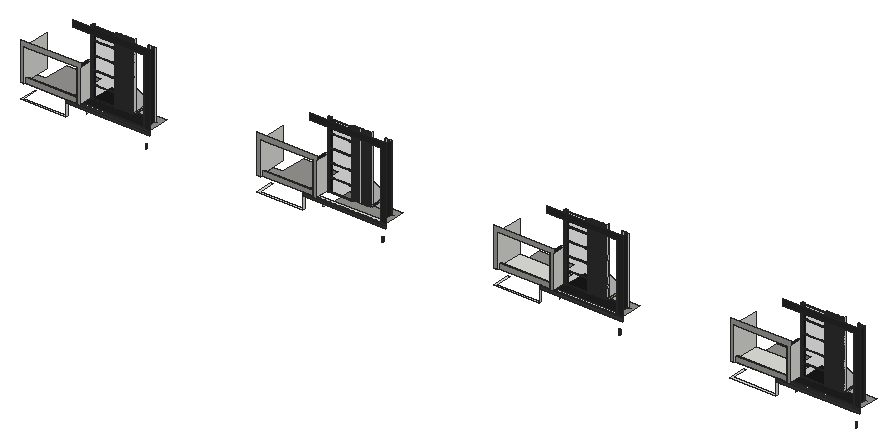
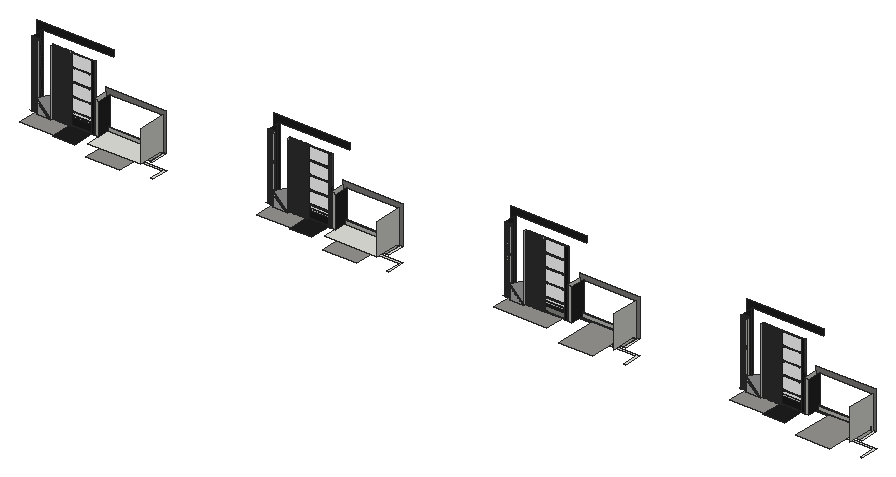
# SketchUp Ruby script. Lengths in inches.
U = 1.inch
M = Sketchup.active_model
def pt(a) = Geom::Point3d.new(a.map { |v| v * U })
def face(e, loops, mat)
  f = e.add_face(loops[0].map { |a| pt(a) })
  loops[1..].each { |l| e.add_face(l.map { |a| pt(a) }).erase! }
  f.material = f.back_material = mat if mat
  f
end
# faces: each face lists its corners as indices into pts; further lists are holes
def faces(e, pts, list, mat = nil) = list.each { |f| face(e, (f[0].is_a?(Array) ? f : [f]).map { |l| l.map { |i| pts[i] } }, mat) }
# xy, xz, yz: faces in a plane at the given z, y or x. An outline is a flat list of corners, or four numbers for a rectangle; further outlines are holes
def ring(l) = l.size == 4 ? [[l[0], l[1]], [l[2], l[1]], [l[2], l[3]], [l[0], l[3]]] : l.each_slice(2).to_a
def flat(e, list, mat, &to3) = list.each { |f| face(e, (f[0].is_a?(Array) ? f : [f]).map { |l| ring(l).map { |u, v| to3.(u, v) } }, mat) }
def xy(e, z, list, mat = nil) = flat(e, list, mat) { |x, y| [x, y, z] }
def xz(e, y, list, mat = nil) = flat(e, list, mat) { |x, z| [x, y, z] }
def yz(e, x, list, mat = nil) = flat(e, list, mat) { |y, z| [x, y, z] }
def lines(e, pts, list) = list.each { |a, b| e.add_line(pt(pts[a]), pt(pts[b])) }
# prism: a flat outline (further loops are holes) pulled along v
def prism(e, loops, v, mat = nil)
  f = face(e, loops, mat); d = Geom::Vector3d.new(v.map { |x| x * U })
  f.pushpull(f.normal.samedirection?(d) ? d.length : -d.length)
end
def box(e, o, s, mat = nil) = prism(e, [[o, [o[0] + s[0], o[1], o[2]], [o[0] + s[0], o[1] + s[1], o[2]], [o[0], o[1] + s[1], o[2]]]], [0, 0, s[2]], mat)
def at(x, y, z, deg = 0) = Geom::Transformation.translation(pt([x, y, z])) * Geom::Transformation.rotation(ORIGIN, Z_AXIS, deg.degrees)
def axes(o, x, y, z) = Geom::Transformation.new([*x, 0, *y, 0, *z, 0, *pt(o).to_a, 1])
def part(name) = M.definitions.add(name)
# library, detail: a bought-in or finely detailed component or shape, given as its bounding box
def library(name, o, s) = part(name).tap { |d| box(d.entities, o, s) }
def detail(e, o, s) = box(e.add_group.entities, o, s)
def put(e, d, t, mat = nil) = e.add_instance(d, t).tap { |i| i.material = mat if mat }
def group(e, t, mat = nil) = e.add_group.tap { |g| g.transformation = t; g.material = mat if mat }.entities
root = M.entities
M.materials.add("Aluminum_Polished").color = [83, 85, 85]
M.materials.add("Glass_Window_Neutral").color = [0, 0, 0]
M.materials["Glass_Window_Neutral"].alpha = 0.125
M.materials.add("[Carrera Marble]").color = [207, 207, 207]
M.materials.add("[Color M07]").color = [58, 58, 58]
M.materials.add("[Color M08]").color = [30, 30, 30]
M.materials.add("[Field Square Tile]").color = [211, 167, 108]
M.materials.add("[Granite Dark Gray]").color = [38, 37, 37]
M.materials.add("[Granite Light Gray]").color = [149, 148, 144]
M.materials.add("[Granite Tile]1").color = [68, 65, 63]
c1 = part("Group\#7")
xy(c1.entities,0,[[6,0,4.45,0.2,3,0.8,1.76,1.76,0.8,3,0.2,4.45,0,6,0.2,7.55,0.8,9,1.76,10.24,3,11.2,4.45,11.8,6,12,7.55,11.8,9,11.2,10.24,10.24,11.2,9,11.8,7.55,12,6,11.8,4.45,11.2,3,10.24,1.76,9,0.8,7.55,0.2]])
xy(c1.entities,37,[[6,0,7.55,0.2,9,0.8,10.24,1.76,11.2,3,11.8,4.45,12,6,11.8,7.55,11.2,9,10.24,10.24,9,11.2,7.55,11.8,6,12,4.45,11.8,3,11.2,1.76,10.24,0.8,9,0.2,7.55,0,6,0.2,4.45,0.8,3,1.76,1.76,3,0.8,4.45,0.2]],"[Granite Tile]1")
p = [[4.45,0.2,0],[6,0,0],[6,0,37],[4.45,0.2,37],[7.55,0.2,0],[7.55,0.2,37],
  [3,0.8,0],[3,0.8,37],[9,0.8,0],[9,0.8,37],[1.76,1.76,0],[1.76,1.76,37],
  [10.24,1.76,0],[10.24,1.76,37],[0.8,3,0],[0.8,3,37],[11.2,3,0],[11.2,3,37],
  [0.2,4.45,0],[0.2,4.45,37],[11.8,4.45,0],[11.8,4.45,37],[0,6,0],[0,6,37],
  [12,6,0],[12,6,37],[0.2,7.55,0],[0.2,7.55,37],[11.8,7.55,0],[11.8,7.55,37],
  [0.8,9,0],[0.8,9,37],[11.2,9,0],[11.2,9,37],[1.76,10.24,0],[1.76,10.24,37],
  [10.24,10.24,0],[10.24,10.24,37],[3,11.2,0],[3,11.2,37],[9,11.2,0],[9,11.2,37],
  [4.45,11.8,0],[4.45,11.8,37],[7.55,11.8,0],[7.55,11.8,37],[6,12,0],[6,12,37]]
faces(c1.entities,p,[[0,1,2,3],[1,4,5,2],[6,0,3,7],[4,8,9,5],[10,6,7,11],[8,12,13,9],[14,10,11,15],[12,16,17,13],
  [18,14,15,19],[16,20,21,17],[22,18,19,23],[20,24,25,21],[26,22,23,27],[24,28,29,25],[30,26,27,31],[28,32,33,29],
  [34,30,31,35],[32,36,37,33],[38,34,35,39],[36,40,41,37],[42,38,39,43],[40,44,45,41],[46,42,43,47],[44,46,47,45]],"[Granite Tile]1")
c2 = part("Group\#54")
box(c2.entities,[0,0,0],[2,1,28])
c3 = part("Group\#56")
p = [[0.11,0.32,0.14],[0.11,0.69,0.14]]
lines(c3.entities,p,[[0,1]])
g1 = group(c3.entities,at(0.11,0,0))
prism(g1,[[[0,0.24,0],[0,0.32,0.14],[0,0.24,0.27],[0,0.08,0.27],[0,0,0.14],[0,0.08,0]]],[-0.11,0,0])
c4 = part("Ver Glass Railing")
g2 = group(c4.entities,at(0,0,0),"Aluminum_Polished")
box(g2,[0,0,0],[2,185,2])
g3 = group(c4.entities,at(0,0,2),"Aluminum_Polished")
p = [[1.41,1,0],[1.41,36.8,0],[1.41,184,0],[1.29,184,0],[1.29,1,0],[1.29,36.8,0],
  [1.41,184,28],[1.29,184,28],[1.41,148.2,28],[1.29,148.2,28],[1.41,1,28],[1.29,1,28],
  [1.29,111.4,28],[1.29,111.4,0],[1.41,111.4,0],[1.41,111.4,28],[1.29,110.4,0],[1.29,110.4,28],
  [1.41,110.4,28],[1.41,110.4,0],[1.29,74.6,28],[1.29,74.6,0],[1.41,74.6,0],[1.41,74.6,28],
  [1.29,73.6,0],[1.29,73.6,28],[1.41,73.6,28],[1.41,73.6,0],[1.29,148.2,0],[1.41,148.2,0],
  [1.29,147.2,0],[1.29,147.2,28],[1.41,147.2,28],[1.41,147.2,0],[1.29,37.8,28],[1.29,37.8,0],
  [1.41,37.8,0],[1.41,37.8,28],[1.29,36.8,28],[1.41,36.8,28]]
lines(g3,p,[[0,1],[2,3],[4,5],[6,7],[6,8],[7,9],[10,11],[2,6],[3,7],[0,4],[11,4],[10,0],
  [12,13],[14,15],[16,17],[18,19],[20,21],[22,23],[24,25],[26,27],[27,22],[24,21],[23,26],[20,25],
  [9,28],[29,8],[30,31],[32,33],[33,29],[30,28],[8,32],[9,31],[34,35],[36,37],[5,38],[39,1],
  [1,36],[5,35],[37,39],[14,33],[19,14],[22,19],[36,27],[13,30],[16,13],[21,16],[35,24],[15,18],
  [12,17],[29,2],[28,3],[18,23],[32,15],[17,20],[31,12],[26,37],[25,34],[34,38],[39,10],[38,11]])
g4 = group(g3,at(1.79,1,0))
box(g4,[-0.5,0,0],[0.125,183,28],"Glass_Window_Neutral")
g5 = group(g3,at(0,184,28))
box(g5,[0,-184,0],[2.5,185,1])
put(g3,c2,axes([2,185,28],[-1,0,0],[0,-1,0],[0,0,-1]))
put(g3,c2,axes([2,1,28],[-1,0,0],[0,-1,0],[0,0,-1]))
put(g3,c2,axes([2,111.4,28],[-1,0,0],[0,-1,0],[0,0,-1]))
put(g3,c2,axes([2,74.6,28],[-1,0,0],[0,-1,0],[0,0,-1]))
g6 = group(g3,at(2,148.2,28))
box(g6,[-2,-1,-28],[2,1,28])
put(g3,c2,axes([2,37.8,28],[-1,0,0],[0,-1,0],[0,0,-1]))
put(g3,c3,at(1.17,146.31,24.26))
put(g3,c3,axes([1.17,148.89,24.54],[1,0,0],[0,-1,0],[0,0,-1]))
put(g3,c3,axes([1.17,148.89,4.79],[1,0,0],[0,-1,0],[0,0,-1]))
put(g3,c3,at(1.17,146.31,4.51))
put(g3,c3,at(1.17,109.51,4.51))
put(g3,c3,axes([1.17,112.09,4.79],[1,0,0],[0,-1,0],[0,0,-1]))
put(g3,c3,axes([1.17,112.09,24.54],[1,0,0],[0,-1,0],[0,0,-1]))
put(g3,c3,at(1.17,109.51,24.26))
put(g3,c3,axes([1.17,75.29,24.54],[1,0,0],[0,-1,0],[0,0,-1]))
put(g3,c3,at(1.17,72.71,4.51))
put(g3,c3,axes([1.17,75.29,4.79],[1,0,0],[0,-1,0],[0,0,-1]))
put(g3,c3,at(1.17,72.71,24.26))
put(g3,c3,axes([1.17,38.49,24.54],[1,0,0],[0,-1,0],[0,0,-1]))
put(g3,c3,at(1.17,35.91,4.51))
put(g3,c3,axes([1.17,38.49,4.79],[1,0,0],[0,-1,0],[0,0,-1]))
put(g3,c3,at(1.17,35.91,24.26))
xy(root,72.4375,[[218.97,457.5625,388.78,457.5625,388.78,465.32,225.79,465.32,225.79,523.18,218.97,523.18],[1097.72,457.5625,1267.53,457.5625,1267.53,465.32,1104.54,465.32,1104.54,523.18,1097.72,523.18],[1976.47,457.5625,2146.28,457.5625,2146.28,465.32,1983.29,465.32,1983.29,523.18,1976.47,523.18],[2855.22,457.5625,3025.03,457.5625,3025.03,465.32,2862.04,465.32,2862.04,523.18,2855.22,523.18]])
xy(root,118.38,[[463.7,458.5,481.29,465.32],[1342.45,458.5,1360.04,465.32],[2221.2,458.5,2238.79,465.32],[3099.95,458.5,3117.54,465.32]])
xy(root,118.38,[[481.29,458.5,678.9,561.06],[1360.04,458.5,1557.65,561.06],[2238.79,458.5,2436.4,561.06],[3117.54,458.5,3315.15,561.06]],"[Granite Light Gray]")
xy(root,128.5,[[218.97,458.5,225.79,523.18],[388.78,458.5,399.95,463.25],[399.95,458.5,427.1,463.25],[427.1,458.5,427.1,463.25,399.95,463.25,399.95,465.32,678.9,465.32,678.9,458.5],[1097.72,458.5,1104.54,523.18],
  [1267.53,458.5,1278.7,463.25],[1278.7,458.5,1305.85,463.25],[1305.85,458.5,1305.85,463.25,1278.7,463.25,1278.7,465.32,1557.65,465.32,1557.65,458.5],[1976.47,458.5,1983.29,523.18],[2146.28,458.5,2157.45,463.25],
  [2157.45,458.5,2184.6,463.25],[2184.6,458.5,2184.6,463.25,2157.45,463.25,2157.45,465.32,2436.4,465.32,2436.4,458.5],[2855.22,458.5,2862.04,523.18],[3025.03,458.5,3036.2,463.25],[3036.2,458.5,3063.35,463.25],
  [3063.35,458.5,3063.35,463.25,3036.2,463.25,3036.2,465.32,3315.15,465.32,3315.15,458.5]])
xy(root,128.5,[[228.78,458.5,228.78,523.18,262.66,523.18,262.66,619.06,388.78,619.06,388.78,463.25,232.96,463.25,232.96,458.5],[1107.53,458.5,1107.53,523.18,1141.41,523.18,1141.41,619.06,1267.53,619.06,1267.53,463.25,1111.71,463.25,1111.71,458.5],[1986.28,458.5,1986.28,523.18,2020.16,523.18,2020.16,619.06,2146.28,619.06,2146.28,463.25,1990.46,463.25,1990.46,458.5],[2865.03,458.5,2865.03,523.18,2898.91,523.18,2898.91,619.06,3025.03,619.06,3025.03,463.25,2869.21,463.25,2869.21,458.5]],"[Granite Light Gray]")
xy(root,134.5,[[442.35,458.5,676.54,458.5,676.54,468.31,444.78,468.31,444.78,511.08,442.35,511.08],[1321.1,458.5,1555.29,458.5,1555.29,468.31,1323.53,468.31,1323.53,511.08,1321.1,511.08],[2199.85,458.5,2434.04,458.5,2434.04,468.31,2202.28,468.31,2202.28,511.08,2199.85,511.08],[3078.6,458.5,3312.79,458.5,3312.79,468.31,3081.03,468.31,3081.03,511.08,3078.6,511.08],[1990.46,468.31,2184.6,561.05],
  [2869.21,468.31,3063.35,561.05],[534.46,508.33,539.88,511.08],[541.08,508.33,546.51,511.08],[547.71,508.33,553.13,511.08],[554.33,508.33,559.76,511.08],
  [560.96,508.33,566.38,511.08],[567.58,508.33,573.01,511.08],[574.21,508.33,579.63,511.08],[580.83,508.33,586.26,511.08],[587.46,508.33,592.88,511.08],
  [594.08,508.33,599.51,511.08],[653.06,508.33,658.48,511.08],[659.68,508.33,665.11,511.08],[666.31,508.33,671.73,511.08],[672.56,508.33,676.54,511.08],
  [676.54,508.33,677.98,511.08],[1413.21,508.33,1418.63,511.08],[1419.83,508.33,1425.26,511.08],[1426.46,508.33,1431.88,511.08],[1433.08,508.33,1438.51,511.08],
  [1439.71,508.33,1445.13,511.08],[1446.33,508.33,1451.76,511.08],[1459.58,508.33,1465.01,511.08],[1466.21,508.33,1471.63,511.08],[1472.83,508.33,1478.26,511.08],
  [1531.81,508.33,1537.23,511.08],[1538.43,508.33,1543.86,511.08],[1545.06,508.33,1550.48,511.08],[1555.29,508.33,1556.73,511.08],[2291.96,508.33,2297.38,511.08],
  [2298.58,508.33,2304.01,511.08],[2305.21,508.33,2310.63,511.08],[2311.83,508.33,2317.26,511.08],[2318.46,508.33,2323.88,511.08],[2325.08,508.33,2330.51,511.08],
  [2331.71,508.33,2337.13,511.08],[2338.33,508.33,2343.76,511.08],[2344.96,508.33,2350.38,511.08],[2351.58,508.33,2357.01,511.08],[2410.56,508.33,2415.98,511.08],
  [2417.18,508.33,2422.61,511.08],[2423.81,508.33,2429.23,511.08],[2430.06,508.33,2434.04,511.08],[2434.04,508.33,2435.48,511.08],[3170.71,508.33,3176.13,511.08],
  [3177.33,508.33,3182.76,511.08],[3183.96,508.33,3189.38,511.08],[3190.58,508.33,3196.01,511.08],[3197.21,508.33,3202.63,511.08],[3203.83,508.33,3209.26,511.08],
  [3210.46,508.33,3215.88,511.08],[3217.08,508.33,3222.51,511.08],[3223.71,508.33,3229.13,511.08],[3230.33,508.33,3235.76,511.08],[3289.31,508.33,3294.73,511.08],
  [3295.93,508.33,3301.36,511.08],[3302.56,508.33,3307.98,511.08],[3308.81,508.33,3312.79,511.08],[3312.79,508.33,3314.23,511.08]])
xy(root,134.5,[[444.78,468.31,676.54,468.31,676.54,508.33,672.56,508.33,672.56,511.08,671.73,511.08,671.73,508.33,666.31,508.33,666.31,511.08,665.11,511.08,665.11,508.33,659.68,508.33,659.68,511.08,658.48,511.08,658.48,508.33,653.06,508.33,653.06,518.65,605.1875,518.65,605.1875,513.52,599.51,513.52,599.51,508.33,594.08,508.33,594.08,511.08,592.88,511.08,592.88,508.33,587.46,508.33,587.46,511.08,586.26,511.08,586.26,508.33,580.83,508.33,580.83,511.08,579.63,511.08,579.63,508.33,574.21,508.33,574.21,511.08,573.01,511.08,573.01,508.33,567.58,508.33,567.58,511.08,566.38,511.08,566.38,508.33,560.96,508.33,560.96,511.08,559.76,511.08,559.76,508.33,554.33,508.33,554.33,511.08,553.13,511.08,553.13,508.33,547.71,508.33,547.71,511.08,546.51,511.08,546.51,508.33,541.08,508.33,541.08,511.08,539.88,511.08,539.88,508.33,534.46,508.33,534.46,589.83,453.7,589.83,453.7,511.08,444.78,511.08],[2202.28,468.31,2434.04,468.31,2434.04,508.33,2430.06,508.33,2430.06,511.08,2429.23,511.08,2429.23,508.33,2423.81,508.33,2423.81,511.08,2422.61,511.08,2422.61,508.33,2417.18,508.33,2417.18,511.08,2415.98,511.08,2415.98,508.33,2410.56,508.33,2410.56,518.65,2362.6875,518.65,2362.6875,513.52,2357.01,513.52,2357.01,508.33,2351.58,508.33,2351.58,511.08,2350.38,511.08,2350.38,508.33,2344.96,508.33,2344.96,511.08,2343.76,511.08,2343.76,508.33,2338.33,508.33,2338.33,511.08,2337.13,511.08,2337.13,508.33,2331.71,508.33,2331.71,511.08,2330.51,511.08,2330.51,508.33,2325.08,508.33,2325.08,511.08,2323.88,511.08,2323.88,508.33,2318.46,508.33,2318.46,511.08,2317.26,511.08,2317.26,508.33,2311.83,508.33,2311.83,511.08,2310.63,511.08,2310.63,508.33,2305.21,508.33,2305.21,511.08,2304.01,511.08,2304.01,508.33,2298.58,508.33,2298.58,511.08,2297.38,511.08,2297.38,508.33,2291.96,508.33,2291.96,589.83,2211.2,589.83,2211.2,511.08,2202.28,511.08],[3081.03,468.31,3312.79,468.31,3312.79,508.33,3308.81,508.33,3308.81,511.08,3307.98,511.08,3307.98,508.33,3302.56,508.33,3302.56,511.08,3301.36,511.08,3301.36,508.33,3295.93,508.33,3295.93,511.08,3294.73,511.08,3294.73,508.33,3289.31,508.33,3289.31,518.65,3241.4375,518.65,3241.4375,513.52,3235.76,513.52,3235.76,508.33,3230.33,508.33,3230.33,511.08,3229.13,511.08,3229.13,508.33,3223.71,508.33,3223.71,511.08,3222.51,511.08,3222.51,508.33,3217.08,508.33,3217.08,511.08,3215.88,511.08,3215.88,508.33,3210.46,508.33,3210.46,511.08,3209.26,511.08,3209.26,508.33,3203.83,508.33,3203.83,511.08,3202.63,511.08,3202.63,508.33,3197.21,508.33,3197.21,511.08,3196.01,511.08,3196.01,508.33,3190.58,508.33,3190.58,511.08,3189.38,511.08,3189.38,508.33,3183.96,508.33,3183.96,511.08,3182.76,511.08,3182.76,508.33,3177.33,508.33,3177.33,511.08,3176.13,511.08,3176.13,508.33,3170.71,508.33,3170.71,589.83,3089.95,589.83,3089.95,511.08,3081.03,511.08]],"[Color M08]")
xz(root,458.5,[[388.78,118.38,698.16,128.5],[1267.53,118.38,1576.91,128.5],[2146.28,118.38,2455.66,128.5],[3025.03,118.38,3334.41,128.5],[442.35,128.5,698.16,134.5],
  [1321.1,128.5,1576.91,134.5],[2199.85,128.5,2455.66,134.5],[3078.6,128.5,3334.41,134.5]],"[Color M07]")
xz(root,458.5,[[676.54,134.5,698.16,134.5,698.16,403.8125,414.98,403.8125,414.98,380.5,676.54,380.5],[1555.29,134.5,1576.91,134.5,1576.91,403.8125,1293.73,403.8125,1293.73,380.5,1555.29,380.5],[2434.04,134.5,2455.66,134.5,2455.66,403.8125,2172.48,403.8125,2172.48,380.5,2434.04,380.5],[3312.79,134.5,3334.41,134.5,3334.41,403.8125,3051.23,403.8125,3051.23,380.5,3312.79,380.5]],"[Granite Dark Gray]")
xz(root,458.5,[[218.97,128.5,232.96,128.5,232.96,251.5,427.1,251.5,427.1,128.5,442.35,128.5,442.35,270.8125,218.97,270.8125],[1097.72,128.5,1111.71,128.5,1111.71,251.5,1305.85,251.5,1305.85,128.5,1321.1,128.5,1321.1,270.8125,1097.72,270.8125],[1976.47,128.5,1990.46,128.5,1990.46,251.5,2184.6,251.5,2184.6,128.5,2199.85,128.5,2199.85,270.8125,1976.47,270.8125],[2855.22,128.5,2869.21,128.5,2869.21,251.5,3063.35,251.5,3063.35,128.5,3078.6,128.5,3078.6,270.8125,2855.22,270.8125]],"[Granite Light Gray]")
xz(root,463.25,[[232.96,128.5,427.1,147.6875],[1111.71,128.5,1305.85,147.6875],[1990.46,128.5,2184.6,147.6875],[2869.21,128.5,3063.35,147.6875]],"[Granite Light Gray]")
xz(root,468.31,[[232.96,134.5,427.1,147.6875],[1111.71,134.5,1305.85,147.6875],[1990.46,134.5,2184.6,147.6875],[2869.21,134.5,3063.35,147.6875]])
xz(root,508.33,[[672.56,134.5,677.98,380.5],[2430.06,134.5,2435.48,380.5],[3308.81,134.5,3314.23,380.5]],"[Field Square Tile]")
xz(root,508.33,[[534.46,134.5,539.88,380.5],[541.08,134.5,546.51,380.5],[547.71,134.5,553.13,380.5],[554.33,134.5,559.76,380.5],[560.96,134.5,566.38,380.5],
  [567.58,134.5,573.01,380.5],[574.21,134.5,579.63,380.5],[580.83,134.5,586.26,380.5],[587.46,134.5,592.88,380.5],[594.08,134.5,599.51,380.5],
  [653.06,134.5,658.48,380.5],[659.68,134.5,665.11,210.79],[666.31,134.5,671.73,380.5],[1413.21,134.5,1418.63,380.5],[1419.83,134.5,1425.26,380.5],
  [1426.46,134.5,1431.88,380.5],[1433.08,134.5,1438.51,380.5],[1446.33,134.5,1451.76,380.5],[1452.96,134.5,1458.38,380.5],[1459.58,134.5,1465.01,380.5],
  [1466.21,134.5,1471.63,380.5],[1472.83,134.5,1478.26,380.5],[1531.81,134.5,1537.23,380.5],[1538.43,134.5,1543.86,210.79],[2291.96,134.5,2297.38,380.5],
  [2298.58,134.5,2304.01,380.5],[2305.21,134.5,2310.63,380.5],[2311.83,134.5,2317.26,380.5],[2318.46,134.5,2323.88,380.5],[2325.08,134.5,2330.51,380.5],
  [2331.71,134.5,2337.13,380.5],[2338.33,134.5,2343.76,380.5],[2344.96,134.5,2350.38,380.5],[2351.58,134.5,2357.01,380.5],[2410.56,134.5,2415.98,380.5],
  [2417.18,134.5,2422.61,210.79],[2423.81,134.5,2429.23,380.5],[3170.71,134.5,3176.13,380.5],[3177.33,134.5,3182.76,380.5],[3183.96,134.5,3189.38,380.5],
  [3190.58,134.5,3196.01,380.5],[3197.21,134.5,3202.63,380.5],[3203.83,134.5,3209.26,380.5],[3210.46,134.5,3215.88,380.5],[3217.08,134.5,3222.51,380.5],
  [3223.71,134.5,3229.13,380.5],[3230.33,134.5,3235.76,380.5],[3289.31,134.5,3294.73,380.5],[3295.93,134.5,3301.36,210.79],[3302.56,134.5,3307.98,380.5]],"[Granite Dark Gray]")
xz(root,511.08,[[427.1,134.5,442.35,134.5,442.35,254.5,433.97,254.5,433.97,251.5,427.1,251.5],[534.46,134.5,539.88,380.5],[539.88,134.5,541.08,380.5],[541.08,134.5,546.51,380.5],[546.51,134.5,547.71,380.5],
  [547.71,134.5,553.13,380.5],[553.13,134.5,554.33,380.5],[554.33,134.5,559.76,380.5],[559.76,134.5,560.96,380.5],[560.96,134.5,566.38,380.5],
  [566.38,134.5,567.58,380.5],[567.58,134.5,573.01,380.5],[573.01,134.5,574.21,380.5],[574.21,134.5,579.63,380.5],[579.63,134.5,580.83,380.5],
  [580.83,134.5,586.26,380.5],[586.26,134.5,587.46,380.5],[587.46,134.5,592.88,380.5],[592.88,134.5,594.08,380.5],[594.08,134.5,599.16,380.5],
  [599.16,134.5,599.51,380.5],[653.06,134.5,658.48,380.5],[658.48,134.5,659.68,380.5],[659.68,134.5,665.11,380.5],[665.11,134.5,666.31,380.5],
  [666.31,134.5,671.73,380.5],[671.73,134.5,672.56,380.5],[672.56,134.5,676.54,380.5],[676.54,134.5,677.98,254.5],[1305.85,134.5,1321.1,134.5,1321.1,254.5,1312.72,254.5,1312.72,251.5,1305.85,251.5],
  [1413.21,134.5,1418.63,380.5],[1418.63,134.5,1419.83,380.5],[1419.83,134.5,1425.26,380.5],[1425.26,134.5,1426.46,380.5],[1426.46,134.5,1431.88,380.5],
  [1431.88,134.5,1433.08,380.5],[1438.51,134.5,1439.71,380.5],[1439.71,134.5,1445.13,380.5],[1445.13,134.5,1446.33,380.5],[1446.33,134.5,1451.76,380.5],
  [1451.76,134.5,1452.96,380.5],[1452.96,134.5,1458.38,380.5],[1458.38,134.5,1459.58,380.5],[1459.58,134.5,1465.01,380.5],[1465.01,134.5,1466.21,380.5],
  [1466.21,134.5,1471.63,380.5],[1471.63,134.5,1472.83,380.5],[1472.83,134.5,1477.91,380.5],[1477.91,134.5,1478.26,380.5],[1543.86,134.5,1545.06,380.5],
  [1545.06,134.5,1550.48,380.5],[1550.48,134.5,1551.31,380.5],[1551.31,134.5,1555.29,380.5],[1555.29,134.5,1556.73,254.5],[2184.6,134.5,2199.85,134.5,2199.85,254.5,2191.47,254.5,2191.47,251.5,2184.6,251.5],
  [2291.96,134.5,2297.38,380.5],[2297.38,134.5,2298.58,380.5],[2298.58,134.5,2304.01,380.5],[2304.01,134.5,2305.21,380.5],[2305.21,134.5,2310.63,380.5],
  [2310.63,134.5,2311.83,380.5],[2311.83,134.5,2317.26,380.5],[2317.26,134.5,2318.46,380.5],[2318.46,134.5,2323.88,380.5],[2323.88,134.5,2325.08,380.5],
  [2325.08,134.5,2330.51,380.5],[2330.51,134.5,2331.71,380.5],[2331.71,134.5,2337.13,380.5],[2337.13,134.5,2338.33,380.5],[2338.33,134.5,2343.76,380.5],
  [2343.76,134.5,2344.96,380.5],[2344.96,134.5,2350.38,380.5],[2350.38,134.5,2351.58,380.5],[2351.58,134.5,2356.66,380.5],[2356.66,134.5,2357.01,380.5],
  [2410.56,134.5,2415.98,380.5],[2415.98,134.5,2417.18,380.5],[2417.18,134.5,2422.61,380.5],[2422.61,134.5,2423.81,380.5],[2423.81,134.5,2429.23,380.5],
  [2429.23,134.5,2430.06,380.5],[2430.06,134.5,2434.04,380.5],[2434.04,134.5,2435.48,254.5],[3063.35,134.5,3078.6,134.5,3078.6,254.5,3070.22,254.5,3070.22,251.5,3063.35,251.5],[3170.71,134.5,3176.13,380.5],
  [3176.13,134.5,3177.33,380.5],[3177.33,134.5,3182.76,380.5],[3182.76,134.5,3183.96,380.5],[3183.96,134.5,3189.38,380.5],[3189.38,134.5,3190.58,380.5],
  [3190.58,134.5,3196.01,380.5],[3196.01,134.5,3197.21,380.5],[3197.21,134.5,3202.63,380.5],[3202.63,134.5,3203.83,380.5],[3203.83,134.5,3209.26,380.5],
  [3209.26,134.5,3210.46,380.5],[3210.46,134.5,3215.88,380.5],[3215.88,134.5,3217.08,380.5],[3217.08,134.5,3222.51,380.5],[3222.51,134.5,3223.71,380.5],
  [3223.71,134.5,3229.13,380.5],[3229.13,134.5,3230.33,380.5],[3230.33,134.5,3235.41,380.5],[3235.41,134.5,3235.76,380.5],[3289.31,134.5,3294.73,380.5],
  [3294.73,134.5,3295.93,380.5],[3295.93,134.5,3301.36,380.5],[3301.36,134.5,3302.56,380.5],[3302.56,134.5,3307.98,380.5],[3307.98,134.5,3308.81,380.5],
  [3308.81,134.5,3312.79,380.5],[3312.79,134.5,3314.23,254.5]])
xz(root,511.08,[[442.35,134.5,453.7,134.5,453.7,380.5,444.78,380.5,444.78,270.8125,442.35,270.8125],[1321.1,134.5,1332.45,134.5,1332.45,380.5,1323.53,380.5,1323.53,270.8125,1321.1,270.8125],[2199.85,134.5,2211.2,134.5,2211.2,380.5,2202.28,380.5,2202.28,270.8125,2199.85,270.8125],[3078.6,134.5,3089.95,134.5,3089.95,380.5,3081.03,380.5,3081.03,270.8125,3078.6,270.8125]],"[Color M08]")
xz(root,513.52,[[599.51,134.5,605.1875,134.5,653.06,178.84,653.06,188.27],[1478.26,134.5,1483.9375,134.5,1531.81,178.84,1531.81,188.27],[2357.01,134.5,2362.6875,134.5,2410.56,178.84,2410.56,188.27],[3235.76,134.5,3241.4375,134.5,3289.31,178.84,3289.31,188.27]],"[Field Square Tile]")
xz(root,518.65,[[599.51,134.5,653.06,188.27,599.51,215.75],[605.1875,134.5,653.06,134.5,653.06,178.84],[1478.26,134.5,1531.81,188.27,1478.26,215.75],[1483.9375,134.5,1531.81,134.5,1531.81,178.84],[2357.01,134.5,2410.56,188.27,2357.01,215.75],
  [2362.6875,134.5,2410.56,134.5,2410.56,178.84],[3235.76,134.5,3289.31,188.27,3235.76,215.75],[3241.4375,134.5,3289.31,134.5,3289.31,178.84]],"[Carrera Marble]")
yz(root,232.96,[[458.5,128.5,463.25,128.5,463.25,147.6875,468.31,147.6875,468.31,134.5,561.05,134.5,561.05,251.5,458.5,251.5]])
yz(root,388.78,[[458.5,72.4375,465.32,128.5]])
yz(root,427.1,[[458.5,128.5,463.25,147.6875]])
yz(root,427.1,[[468.31,134.5,468.31,147.6875,458.5,147.6875,458.5,251.5,511.08,251.5,511.08,134.5]],"[Granite Dark Gray]")
yz(root,442.35,[[458.5,134.5,511.08,254.5]])
yz(root,463.7,[[458.5,110.32,465.32,118.38]])
yz(root,534.46,[[508.33,134.5,511.08,380.5]])
yz(root,539.88,[[508.33,134.5,511.08,380.5]])
yz(root,541.08,[[508.33,134.5,511.08,380.5]])
yz(root,546.51,[[508.33,134.5,511.08,380.5]])
yz(root,547.71,[[508.33,134.5,511.08,380.5]])
yz(root,553.13,[[508.33,134.5,511.08,380.5]])
yz(root,554.33,[[508.33,134.5,511.08,380.5]])
yz(root,559.76,[[508.33,134.5,511.08,380.5]])
yz(root,560.96,[[508.33,134.5,511.08,380.5]])
yz(root,566.38,[[508.33,134.5,511.08,380.5]])
yz(root,567.58,[[508.33,134.5,511.08,380.5]])
yz(root,573.01,[[508.33,134.5,511.08,380.5]])
yz(root,574.21,[[508.33,134.5,511.08,380.5]])
yz(root,579.63,[[508.33,134.5,511.08,380.5]])
yz(root,580.83,[[508.33,134.5,511.08,380.5]])
yz(root,586.26,[[508.33,134.5,511.08,380.5]])
yz(root,587.46,[[508.33,134.5,511.08,380.5]])
yz(root,592.88,[[508.33,134.5,511.08,380.5]])
yz(root,594.08,[[508.33,134.5,511.08,380.5]])
yz(root,599.51,[[508.33,134.5,511.08,380.5],[511.08,134.5,518.65,380.5]])
yz(root,653.06,[[508.33,134.5,511.08,380.5],[511.08,134.5,511.08,380.5,513.52,380.5,513.52,374,518.65,374,518.65,290.71,513.52,290.71,513.52,275.14,518.65,275.14,518.65,192.89,513.52,192.89,513.52,178.84,518.65,178.84,518.65,134.5]])
yz(root,658.48,[[508.33,134.5,511.08,380.5]])
yz(root,659.68,[[508.33,134.5,508.33,210.79,501.4,210.79,501.4,223.24,508.33,223.24,508.33,282.18,501.4,282.18,501.4,296.03,508.33,296.03,508.33,380.5,511.08,380.5,511.08,134.5]])
yz(root,665.11,[[508.33,134.5,511.08,134.5,511.08,380.5,508.33,380.5,508.33,296.03,501.4,296.03,501.4,282.18,508.33,282.18,508.33,223.24,501.4,223.24,501.4,210.79,508.33,210.79]])
yz(root,666.31,[[508.33,134.5,511.08,380.5]])
yz(root,671.73,[[508.33,134.5,511.08,380.5]])
yz(root,672.56,[[508.33,134.5,511.08,380.5]])
yz(root,676.54,[[458.5,134.5,468.31,380.5],[468.31,134.5,511.08,380.5]],"[Granite Dark Gray]")
yz(root,677.98,[[508.33,134.5,511.08,380.5]])
yz(root,1111.71,[[458.5,128.5,463.25,128.5,463.25,147.6875,468.31,147.6875,468.31,134.5,561.05,134.5,561.05,251.5,458.5,251.5]])
yz(root,1267.53,[[458.5,72.4375,465.32,128.5]])
yz(root,1305.85,[[458.5,128.5,463.25,147.6875]])
yz(root,1305.85,[[468.31,134.5,468.31,147.6875,458.5,147.6875,458.5,251.5,511.08,251.5,511.08,134.5]],"[Granite Dark Gray]")
yz(root,1321.1,[[458.5,134.5,511.08,254.5]])
yz(root,1342.45,[[458.5,110.32,465.32,118.38]])
yz(root,1413.21,[[508.33,134.5,511.08,380.5]])
yz(root,1418.63,[[508.33,134.5,511.08,380.5]])
yz(root,1419.83,[[508.33,134.5,511.08,380.5]])
yz(root,1425.26,[[508.33,134.5,511.08,380.5]])
yz(root,1426.46,[[508.33,134.5,511.08,380.5]])
yz(root,1431.88,[[508.33,134.5,511.08,380.5]])
yz(root,1433.08,[[508.33,134.5,511.08,380.5]])
yz(root,1438.51,[[508.33,134.5,511.08,380.5]])
yz(root,1439.71,[[508.33,134.5,511.08,380.5]])
yz(root,1445.13,[[508.33,134.5,511.08,380.5]])
yz(root,1446.33,[[508.33,134.5,511.08,380.5]])
yz(root,1451.76,[[508.33,134.5,511.08,380.5]])
yz(root,1452.96,[[508.33,134.5,511.08,380.5]])
yz(root,1458.38,[[508.33,134.5,511.08,380.5]])
yz(root,1459.58,[[508.33,134.5,511.08,380.5]])
yz(root,1465.01,[[508.33,134.5,511.08,380.5]])
yz(root,1466.21,[[508.33,134.5,511.08,380.5]])
yz(root,1471.63,[[508.33,134.5,511.08,380.5]])
yz(root,1472.83,[[508.33,134.5,511.08,380.5]])
yz(root,1478.26,[[508.33,134.5,511.08,380.5],[511.08,134.5,518.65,380.5]])
yz(root,1531.81,[[511.08,134.5,511.08,380.5,513.52,380.5,513.52,374,518.65,374,518.65,290.71,513.52,290.71,513.52,275.14,518.65,275.14,518.65,192.89,513.52,192.89,513.52,178.84,518.65,178.84,518.65,134.5]])
yz(root,1537.23,[[508.33,134.5,511.08,380.5]])
yz(root,1551.31,[[508.33,134.5,511.08,380.5]])
yz(root,1555.29,[[468.31,134.5,511.08,380.5]],"[Granite Dark Gray]")
yz(root,1556.73,[[508.33,134.5,511.08,380.5]])
yz(root,1990.46,[[458.5,128.5,463.25,128.5,463.25,147.6875,468.31,147.6875,468.31,134.5,561.05,134.5,561.05,251.5,458.5,251.5]])
yz(root,2146.28,[[458.5,72.4375,465.32,128.5]])
yz(root,2184.6,[[458.5,128.5,463.25,147.6875]])
yz(root,2184.6,[[468.31,134.5,468.31,147.6875,458.5,147.6875,458.5,251.5,511.08,251.5,511.08,134.5]],"[Granite Dark Gray]")
yz(root,2199.85,[[458.5,134.5,511.08,254.5]])
yz(root,2221.2,[[458.5,110.32,465.32,118.38]])
yz(root,2291.96,[[508.33,134.5,511.08,380.5]])
yz(root,2297.38,[[508.33,134.5,511.08,380.5]])
yz(root,2298.58,[[508.33,134.5,511.08,380.5]])
yz(root,2304.01,[[508.33,134.5,511.08,380.5]])
yz(root,2305.21,[[508.33,134.5,511.08,380.5]])
yz(root,2310.63,[[508.33,134.5,511.08,380.5]])
yz(root,2311.83,[[508.33,134.5,511.08,380.5]])
yz(root,2317.26,[[508.33,134.5,511.08,380.5]])
yz(root,2318.46,[[508.33,134.5,511.08,380.5]])
yz(root,2323.88,[[508.33,134.5,511.08,380.5]])
yz(root,2325.08,[[508.33,134.5,511.08,380.5]])
yz(root,2330.51,[[508.33,134.5,511.08,380.5]])
yz(root,2331.71,[[508.33,134.5,511.08,380.5]])
yz(root,2337.13,[[508.33,134.5,511.08,380.5]])
yz(root,2338.33,[[508.33,134.5,511.08,380.5]])
yz(root,2343.76,[[508.33,134.5,511.08,380.5]])
yz(root,2344.96,[[508.33,134.5,511.08,380.5]])
yz(root,2350.38,[[508.33,134.5,511.08,380.5]])
yz(root,2351.58,[[508.33,134.5,511.08,380.5]])
yz(root,2357.01,[[508.33,134.5,511.08,380.5],[511.08,134.5,518.65,380.5]])
yz(root,2410.56,[[508.33,134.5,511.08,380.5],[511.08,134.5,511.08,380.5,513.52,380.5,513.52,374,518.65,374,518.65,290.71,513.52,290.71,513.52,275.14,518.65,275.14,518.65,192.89,513.52,192.89,513.52,178.84,518.65,178.84,518.65,134.5]])
yz(root,2415.98,[[508.33,134.5,511.08,380.5]])
yz(root,2417.18,[[508.33,134.5,508.33,210.79,501.4,210.79,501.4,223.24,508.33,223.24,508.33,282.18,501.4,282.18,501.4,296.03,508.33,296.03,508.33,380.5,511.08,380.5,511.08,134.5]])
yz(root,2422.61,[[508.33,134.5,511.08,134.5,511.08,380.5,508.33,380.5,508.33,296.03,501.4,296.03,501.4,282.18,508.33,282.18,508.33,223.24,501.4,223.24,501.4,210.79,508.33,210.79]])
yz(root,2423.81,[[508.33,134.5,511.08,380.5]])
yz(root,2429.23,[[508.33,134.5,511.08,380.5]])
yz(root,2430.06,[[508.33,134.5,511.08,380.5]])
yz(root,2434.04,[[458.5,134.5,468.31,380.5],[468.31,134.5,511.08,380.5]],"[Granite Dark Gray]")
yz(root,2435.48,[[508.33,134.5,511.08,380.5]])
yz(root,2869.21,[[458.5,128.5,463.25,128.5,463.25,147.6875,468.31,147.6875,468.31,134.5,561.05,134.5,561.05,251.5,458.5,251.5]])
yz(root,3025.03,[[458.5,72.4375,465.32,128.5]])
yz(root,3063.35,[[458.5,128.5,463.25,147.6875]])
yz(root,3063.35,[[468.31,134.5,468.31,147.6875,458.5,147.6875,458.5,251.5,511.08,251.5,511.08,134.5]],"[Granite Dark Gray]")
yz(root,3078.6,[[458.5,134.5,511.08,254.5]])
yz(root,3099.95,[[458.5,110.32,465.32,118.38]])
yz(root,3170.71,[[508.33,134.5,511.08,380.5]])
yz(root,3176.13,[[508.33,134.5,511.08,380.5]])
yz(root,3177.33,[[508.33,134.5,511.08,380.5]])
yz(root,3182.76,[[508.33,134.5,511.08,380.5]])
yz(root,3183.96,[[508.33,134.5,511.08,380.5]])
yz(root,3189.38,[[508.33,134.5,511.08,380.5]])
yz(root,3190.58,[[508.33,134.5,511.08,380.5]])
yz(root,3196.01,[[508.33,134.5,511.08,380.5]])
yz(root,3197.21,[[508.33,134.5,511.08,380.5]])
yz(root,3202.63,[[508.33,134.5,511.08,380.5]])
yz(root,3203.83,[[508.33,134.5,511.08,380.5]])
yz(root,3209.26,[[508.33,134.5,511.08,380.5]])
yz(root,3210.46,[[508.33,134.5,511.08,380.5]])
yz(root,3215.88,[[508.33,134.5,511.08,380.5]])
yz(root,3217.08,[[508.33,134.5,511.08,380.5]])
yz(root,3222.51,[[508.33,134.5,511.08,380.5]])
yz(root,3223.71,[[508.33,134.5,511.08,380.5]])
yz(root,3229.13,[[508.33,134.5,511.08,380.5]])
yz(root,3230.33,[[508.33,134.5,511.08,380.5]])
yz(root,3235.76,[[508.33,134.5,511.08,380.5],[511.08,134.5,518.65,380.5]])
yz(root,3289.31,[[508.33,134.5,511.08,380.5],[511.08,134.5,511.08,380.5,513.52,380.5,513.52,374,518.65,374,518.65,290.71,513.52,290.71,513.52,275.14,518.65,275.14,518.65,192.89,513.52,192.89,513.52,178.84,518.65,178.84,518.65,134.5]])
yz(root,3294.73,[[508.33,134.5,511.08,380.5]])
yz(root,3295.93,[[508.33,134.5,508.33,210.79,501.4,210.79,501.4,223.24,508.33,223.24,508.33,282.18,501.4,282.18,501.4,296.03,508.33,296.03,508.33,380.5,511.08,380.5,511.08,134.5]])
yz(root,3301.36,[[508.33,134.5,511.08,134.5,511.08,380.5,508.33,380.5,508.33,296.03,501.4,296.03,501.4,282.18,508.33,282.18,508.33,223.24,501.4,223.24,501.4,210.79,508.33,210.79]])
yz(root,3302.56,[[508.33,134.5,511.08,380.5]])
yz(root,3307.98,[[508.33,134.5,511.08,380.5]])
yz(root,3308.81,[[508.33,134.5,511.08,380.5]])
yz(root,3312.79,[[458.5,134.5,468.31,380.5],[468.31,134.5,511.08,380.5]],"[Granite Dark Gray]")
yz(root,3314.23,[[508.33,134.5,511.08,380.5]])
p = [[653.06,518.65,188.27],[599.51,518.65,134.5],[599.51,513.52,134.5],[653.06,513.52,188.27],[605.1875,518.65,134.5],[653.06,518.65,178.84],
  [653.06,513.52,178.84],[605.1875,513.52,134.5],[1531.81,518.65,188.27],[1478.26,518.65,134.5],[1478.26,513.52,134.5],[1531.81,513.52,188.27],
  [1483.9375,518.65,134.5],[1531.81,518.65,178.84],[1531.81,513.52,178.84],[1483.9375,513.52,134.5],[2410.56,518.65,188.27],[2357.01,518.65,134.5],
  [2357.01,513.52,134.5],[2410.56,513.52,188.27],[2362.6875,518.65,134.5],[2410.56,518.65,178.84],[2410.56,513.52,178.84],[2362.6875,513.52,134.5],
  [3289.31,518.65,188.27],[3235.76,518.65,134.5],[3235.76,513.52,134.5],[3289.31,513.52,188.27],[3241.4375,518.65,134.5],[3289.31,518.65,178.84],
  [3289.31,513.52,178.84],[3241.4375,513.52,134.5],[2436.4,465.32,118.38],[2436.4,465.32,128.5],[2435.48,511.08,134.5],[2443.85,511.08,134.5],
  [3315.15,465.32,118.38],[3315.15,465.32,128.5],[3314.23,511.08,134.5],[3322.6,511.08,134.5],[678.9,465.32,118.38],[678.9,465.32,128.5],
  [677.98,511.08,134.5],[686.35,511.08,134.5],[1557.65,465.32,118.38],[1557.65,465.32,128.5],[1556.73,511.08,134.5],[1565.1,511.08,134.5]]
faces(root,p,[[0,1,2,3],[4,5,6,7],[8,9,10,11],[12,13,14,15],[16,17,18,19],[20,21,22,23],[24,25,26,27],[28,29,30,31]])
lines(root,p,[[32,33],[34,35],[36,37],[38,39],[40,41],[42,43],[44,45],[46,47]])
put(root,c1,axes([2443.36,453.46,72.9375],[0.42,0,0],[0,0.42,0],[0,0,0.42]))
put(root,c1,axes([3322.11,453.46,72.9375],[0.42,0,0],[0,0.42,0],[0,0,0.42]))
put(root,c1,axes([685.86,453.46,72.9375],[0.42,0,0],[0,0.42,0],[0,0,0.42]))
put(root,c1,axes([1564.61,453.46,72.9375],[0.42,0,0],[0,0.42,0],[0,0,0.42]))
put(root,c4,axes([2201.18,505.01,132.28],[0,1.33,0],[0,0,1.33],[2.92826,0,0]),"[Granite Dark Gray]")
put(root,c4,axes([3079.93,505.01,132.28],[0,1.33,0],[0,0,1.33],[2.92826,0,0]),"[Granite Dark Gray]")
put(root,c4,axes([443.68,505.01,132.28],[0,1.33,0],[0,0,1.33],[2.92826,0,0]),"[Granite Dark Gray]")
put(root,c4,axes([1322.43,505.01,132.28],[0,1.33,0],[0,0,1.33],[2.92826,0,0]),"[Granite Dark Gray]")
